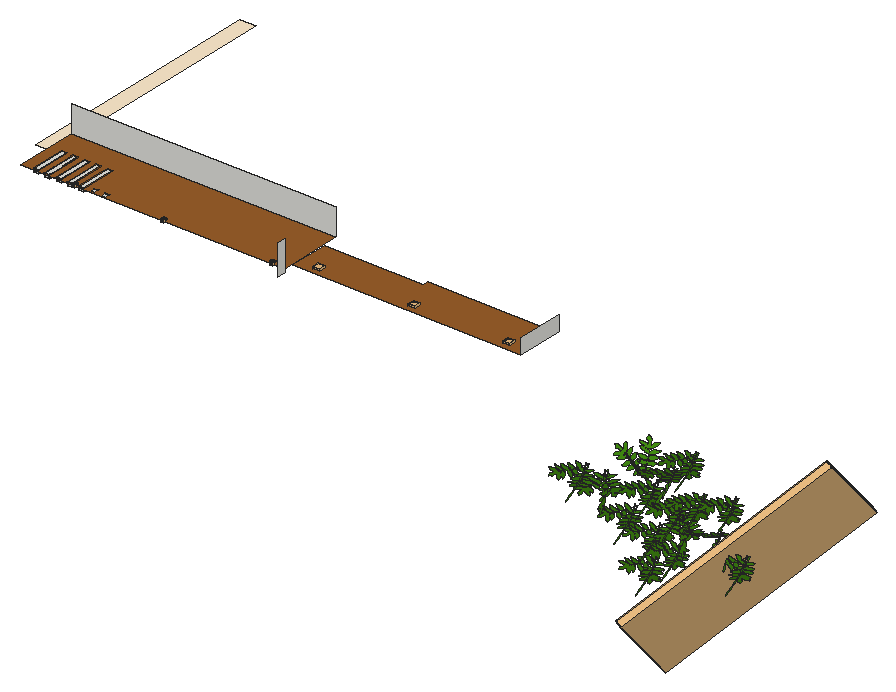
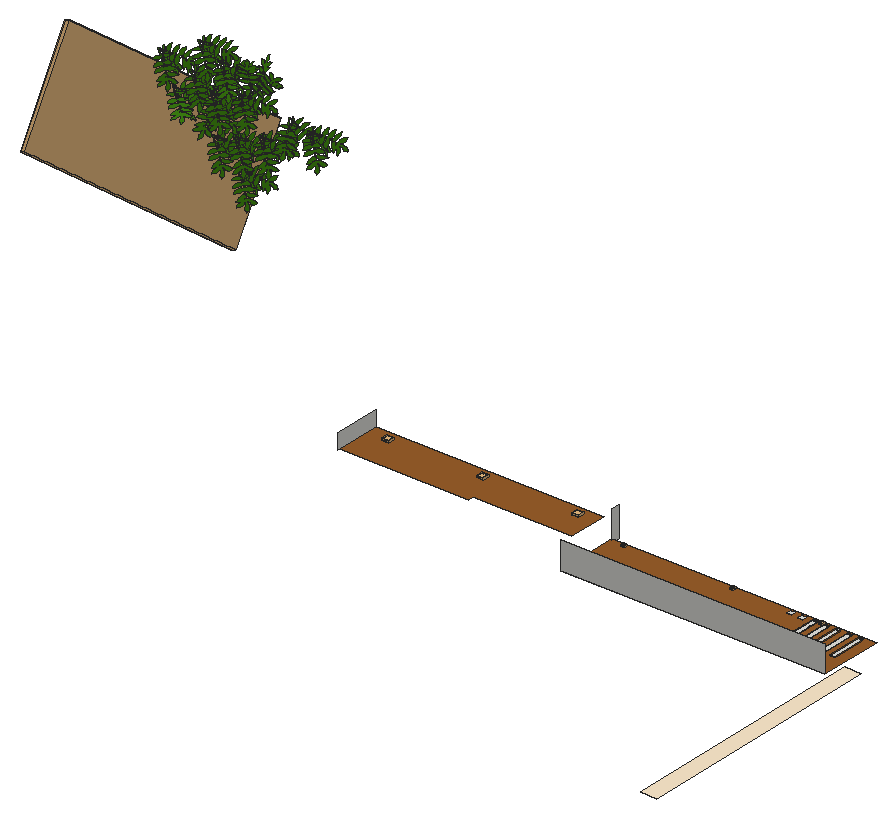
# SketchUp Ruby script. Lengths in inches.
U = 1.inch
M = Sketchup.active_model
def pt(a) = Geom::Point3d.new(a.map { |v| v * U })
def face(e, loops, mat)
  f = e.add_face(loops[0].map { |a| pt(a) })
  loops[1..].each { |l| e.add_face(l.map { |a| pt(a) }).erase! }
  f.material = f.back_material = mat if mat
  f
end
# faces: each face lists its corners as indices into pts; further lists are holes
def faces(e, pts, list, mat = nil) = list.each { |f| face(e, (f[0].is_a?(Array) ? f : [f]).map { |l| l.map { |i| pts[i] } }, mat) }
# xy, xz, yz: faces in a plane at the given z, y or x. An outline is a flat list of corners, or four numbers for a rectangle; further outlines are holes
def ring(l) = l.size == 4 ? [[l[0], l[1]], [l[2], l[1]], [l[2], l[3]], [l[0], l[3]]] : l.each_slice(2).to_a
def flat(e, list, mat, &to3) = list.each { |f| face(e, (f[0].is_a?(Array) ? f : [f]).map { |l| ring(l).map { |u, v| to3.(u, v) } }, mat) }
def xy(e, z, list, mat = nil) = flat(e, list, mat) { |x, y| [x, y, z] }
def xz(e, y, list, mat = nil) = flat(e, list, mat) { |x, z| [x, y, z] }
def yz(e, x, list, mat = nil) = flat(e, list, mat) { |y, z| [x, y, z] }
def lines(e, pts, list) = list.each { |a, b| e.add_line(pt(pts[a]), pt(pts[b])) }
# prism: a flat outline (further loops are holes) pulled along v
def prism(e, loops, v, mat = nil)
  f = face(e, loops, mat); d = Geom::Vector3d.new(v.map { |x| x * U })
  f.pushpull(f.normal.samedirection?(d) ? d.length : -d.length)
end
def box(e, o, s, mat = nil) = prism(e, [[o, [o[0] + s[0], o[1], o[2]], [o[0] + s[0], o[1] + s[1], o[2]], [o[0], o[1] + s[1], o[2]]]], [0, 0, s[2]], mat)
def at(x, y, z, deg = 0) = Geom::Transformation.translation(pt([x, y, z])) * Geom::Transformation.rotation(ORIGIN, Z_AXIS, deg.degrees)
def axes(o, x, y, z) = Geom::Transformation.new([*x, 0, *y, 0, *z, 0, *pt(o).to_a, 1])
def part(name) = M.definitions.add(name)
# library, detail: a bought-in or finely detailed component or shape, given as its bounding box
def library(name, o, s) = part(name).tap { |d| box(d.entities, o, s) }
def detail(e, o, s) = box(e.add_group.entities, o, s)
def put(e, d, t, mat = nil) = e.add_instance(d, t).tap { |i| i.material = mat if mat }
def group(e, t, mat = nil) = e.add_group.tap { |g| g.transformation = t; g.material = mat if mat }.entities
root = M.entities
M.materials.add("[0029_BlanchedAlmond]").color = [255, 235, 205]
M.materials.add("[Wood Floor Dark]").color = [153, 94, 42]
M.materials.add("hojas").color = [70, 150, 19]
c1 = library("Group\#88",[0,0,0],[77.52,5,145.33])
c2 = library("A$C06767DEF\#1",[-8.3,1.21,0],[7.09,7.09,5.51])
c3 = part("rama-acacia")
p = [[-13.53,0.69,-1.07],[-13.38,0.86,-0.98],[-13.61,0.85,-1.06],[-14.07,0.85,-1.21],[-15.17,0.86,-1.58],[-15.95,0.92,-1.83],
  [-16.01,1,-1.83],[-16.01,1.17,-1.78],[-16.07,1.93,-1.6],[-16.4,2.73,-1.5],[-16.65,3.06,-1.5],[-17.13,4.01,-1.41],
  [-17.78,4.7,-1.44],[-18.28,5.07,-1.51],[-18.57,5.18,-1.58],[-18.91,5.47,-1.62],[-19.07,5.48,-1.67],[-19.35,5.61,-1.73],
  [-19.51,5.64,-1.78],[-19.38,5.57,-1.75],[-19.33,5.5,-1.75],[-19.31,5.23,-1.82],[-19.38,5.08,-1.89],[-19.41,4.84,-1.96],
  [-19.36,4.59,-2.01],[-19.43,4.55,-2.04],[-19.36,4.15,-2.125],[-19.21,3.7,-2.19],[-18.875,3.1,-2.24],[-18.61,2.78,-2.24],
  [-17.83,2.19,-2.13],[-17.4375,1.85,-2.09],[-17.04,1.49,-2.05],[-16.61,1.24,-1.97],[-16.17,1.0625,-1.87],[-16.06,0.95,-1.86],
  [-16.06,0.91,-1.87],[-16.32,0.9,-1.96],[-16.7,0.88,-2.1],[-17.05,0.91,-2.21],[-17.61,1.15,-2.33],[-18.06,1.29,-2.45],
  [-18.88,1.53,-2.67],[-20.25,1.46,-3.15],[-20.59,1.49,-3.26],[-20.79,1.37,-3.36],[-21.08,1.2,-3.5],[-21.28,1.22,-3.5625],
  [-21.48,0.94,-3.71],[-21.79,0.5,-3.93],[-22.02,0.17,-4.1],[-22.11,0.05,-4.16],[-22.21,-0.02,-4.21],[-22.375,-0.05,-4.28],
  [-22.375,-0.07,-4.28],[-22.18,-0.09,-4.22],[-22.11,-0.07,-4.19],[-21.78,-0.1,-4.09],[-21.6,-0.18,-4.05],[-21.52,-0.27,-4.04],
  [-21.33,-0.33,-4],[-20.94,-0.54,-3.92],[-20.6875,-0.63,-3.86],[-20.54,-0.68,-3.82],[-20.42,-0.67,-3.78],[-20.09,-0.46,-3.61],
  [-19.8,-0.24,-3.45],[-19.21,-0.02,-3.19],[-18.48,0.08,-2.92],[-17.72,0.38,-2.58],[-17.4,0.5,-2.4375],[-16.93,0.75,-2.21],
  [-16.78,0.8,-2.15],[-16.1,0.83,-1.91],[-16.0625,0.81,-1.9],[-16.08,0.77,-1.91],[-16.27,0.72,-1.99],[-16.88,0.39,-2.29],
  [-17.1875,0.15,-2.46],[-17.27,0.02,-2.52],[-17.94,-0.52,-2.89],[-17.94,-0.59,-2.91],[-18.08,-0.68,-2.99],[-18.13,-0.86,-3.05],
  [-18.56,-1.55,-3.38],[-18.71,-2.11,-3.58],[-18.79,-2.61,-3.74],[-18.86,-2.84,-3.83],[-18.87,-3.07,-3.89],[-18.84,-3.22,-3.92],
  [-18.8,-3.26,-3.92],[-18.76,-3.47,-3.96],[-18.76,-3.6,-4],[-18.67,-3.8,-4.02],[-18.61,-3.92,-4.04],[-18.58,-4.11,-4.07],
  [-18.53,-4.18,-4.08],[-18.58,-4.35,-4.14],[-18.65,-4.43,-4.18],[-18.72,-4.51,-4.23],[-18.8125,-4.51,-4.26],[-18.8125,-4.53,-4.26],
  [-18.72,-4.54,-4.24],[-18.66,-4.49,-4.21],[-18.58,-4.43,-4.16],[-18.35,-4.23,-4.03],[-18.32,-4.17,-4],[-18.22,-4.125,-3.95],
  [-18.1,-4,-3.88],[-17.79,-3.72,-3.7],[-17.68,-3.51,-3.61],[-17.32,-3.13,-3.38],[-17.24,-2.94,-3.31],[-16.78,-2.12,-2.93],
  [-16.48,-1.78,-2.73],[-16.3,-1.28,-2.54],[-16.05,-0.75,-2.3125],[-15.89,-0.2,-2.11],[-15.89,0.39,-1.95],[-15.96,0.79,-1.87],
  [-15.91,0.82,-1.84],[-15.27,0.8,-1.63],[-14.18,0.76,-1.27],[-13.78,0.73,-1.15],[-13.78,0.67,-1.16],[-14.23,0.54,-1.35],
  [-14.65,0.33,-1.55],[-14.97,0.02,-1.74],[-15.25,-0.36,-1.9375],[-15.57,-0.72,-2.14],[-15.96,-1.64,-2.52],[-16.2,-2.51,-2.84],
  [-16.2,-3.12,-3],[-16.14,-3.41,-3.06],[-16.1,-3.75,-3.14],[-16.1,-4.09,-3.23],[-16.2,-4.25,-3.3],[-16.2,-4.28,-3.3125],
  [-16.08,-4.19,-3.24],[-15.98,-4.08,-3.18],[-15.96,-3.94,-3.14],[-15.96,-3.8125,-3.1],[-15.9,-3.72,-3.06],[-15.68,-3.55,-2.9375],
  [-15.51,-3.49,-2.86],[-15.3,-3.33,-2.75],[-15.23,-3.17,-2.68],[-15.01,-3.03,-2.57],[-14.875,-2.83,-2.47],[-14.6,-2.59,-2.3125],
  [-14.4,-2.27,-2.16],[-14.12,-1.6,-1.89],[-13.91,-1.1,-1.68],[-13.67,-0.83,-1.53],[-13.53,-0.45,-1.38],[-13.53,0.67,-1.08],
  [-12.41,6.01,0.65],[-12.44,6.14,0.68],[-12.41,6.29,0.73],[-12.43,6.29,0.73],[-12.44,6.26,0.72],[-12.47,6.15,0.68],
  [-12.49,6.07,0.66],[-12.57,5.75,0.55],[-12.67,5.36,0.43],[-12.79,4.875,0.28],[-12.83,4.52,0.18],[-12.83,3.99,0.04],
  [-12.73,3.11,-0.18],[-12.58,2.52,-0.3125],[-12.3,1.97,-0.41],[-11.88,1.51,-0.46],[-11.37,1.0625,-0.48],[-10.75,0.75,-0.45],
  [-10.75,0.68,-0.47],[-12.55,0.7,-0.79],[-13.21,0.79,-0.89],[-13.2,0.67,-0.92],[-12.56,0.62,-0.82],[-11.15,0.56,-0.58],
  [-10.79,0.54,-0.52],[-10.72,0.52,-0.51],[-10.72,0.5,-0.52],[-10.87,0.47,-0.55],[-11.14,0.41,-0.62],[-11.39,0.27,-0.7],
  [-11.625,-0.01,-0.82],[-11.8,-0.43,-0.96],[-11.83,-0.57,-1],[-12.02,-1.08,-1.17],[-12.1,-1.39,-1.27],[-12.17,-1.95,-1.4375],
  [-12.17,-2.77,-1.65],[-12.09,-3.59,-1.86],[-11.86,-4.26,-2],[-11.8125,-4.4,-2.03],[-11.84,-4.49,-2.05],[-11.91,-4.6,-2.1],
  [-11.97,-4.65,-2.12],[-11.98,-4.67,-2.13],[-11.92,-4.65,-2.11],[-11.84,-4.59,-2.08],[-11.77,-4.52,-2.05],[-11.74,-4.47,-2.03],
  [-11.37,-4.3125,-1.92],[-10.95,-4.0625,-1.78],[-10.82,-3.89,-1.71],[-10.64,-3.57,-1.59],[-10.41,-3.05,-1.41],[-10.27,-2.73,-1.3],
  [-10.07,-1.88,-1.03],[-10.15,-0.71,-0.73],[-10.31,-0.1,-0.6],[-10.5,0.4,-0.5],[-10.5,0.48,-0.48],[-10.44,0.53,-0.45],
  [-10.39,0.64,-0.42],[-10.52,0.73,-0.42],[-10.44,0.93,-0.35],[-10.44,1.2,-0.28],[-10.32,1.47,-0.18],[-10.48,2.6875,0.12],
  [-10.43,2.96,0.2],[-10.75,3.87,0.38],[-11.26,4.93,0.57],[-11.8,5.54,0.64],[-12.37,5.93,0.64],[-7.78,0.19,-0.06],
  [-7.78,0.25,-0.04],[-7.75,0.39,0],[-7.89,0.4,-0.02],[-7.96,0.46,-0.02],[-7.96,0.49,-0.01],[-7.76,0.62,0.06],
  [-7.53,0.99,0.2],[-7.31,1.78,0.45],[-7.31,2.74,0.71],[-7.63,3.6875,0.9],[-8.02,4.57,1.07],[-8.66,5.23,1.13],
  [-8.83,5.4,1.14],[-8.92,5.54,1.16],[-9.1,5.64,1.16],[-9.08,5.6,1.15],[-9.02,5.56,1.15],[-8.94,5.46,1.14],
  [-8.9,5.37,1.12],[-8.9375,5.25,1.08],[-9.14,4.92,0.96],[-9.31,4.5625,0.83],[-9.39,3.73,0.6],[-9.44,2.76,0.32],
  [-9.23,1.59,0.05],[-8.82,0.9,-0.06],[-8.36,0.59,-0.0625],[-8.14,0.51,-0.04],[-8.05,0.48,-0.03],[-8.05,0.46,-0.04],
  [-8.12,0.43,-0.06],[-10.1,0.49,-0.4],[-8.22,0.3125,-0.11],[-8.22,0.25,-0.125],[-8.53,0.13,-0.21],[-8.8,-0.16,-0.34],
  [-8.96,-0.61,-0.49],[-8.96,-0.87,-0.56],[-9.16,-1.42,-0.74],[-9.13,-1.77,-0.83],[-9.09,-1.83,-0.84],[-9.125,-1.92,-0.87],
  [-9.125,-2.13,-0.93],[-9.08,-2.23,-0.95],[-9.15,-2.39,-1],[-9.11,-2.67,-1.07],[-9.03,-2.86,-1.11],[-9.07,-3.03,-1.16],
  [-8.97,-3.23,-1.19],[-8.93,-3.44,-1.24],[-8.93,-3.71,-1.32],[-8.79,-4.05,-1.38],[-8.7,-4.25,-1.42],[-8.7,-4.39,-1.46],
  [-8.76,-4.53,-1.5],[-8.77,-4.65,-1.54],[-8.64,-4.55,-1.49],[-8.27,-4.22,-1.33],[-8.1875,-4.06,-1.27],[-8.07,-3.98,-1.23],
  [-7.98,-3.79,-1.17],[-7.79,-3.59,-1.08],[-7.64,-3.3,-0.97],[-7.64,-3.25,-0.96],[-7.59,-3.21,-0.9375],[-7.52,-2.93,-0.85],
  [-7.52,-2.85,-0.83],[-7.47,-2.81,-0.81],[-7.3,-2.09,-0.59],[-7.32,-2.01,-0.57],[-7.27,-1.95,-0.54],[-7.1875,-1.57,-0.42],
  [-7.17,-1.46,-0.39],[-7.17,-1.16,-0.3125],[-7.23,-0.61,-0.17],[-7.49,-0.15,-0.1],[-13.39,-0.07,-1.23],[-13.39,0.25,-1.14],
  [-13.49,0.5625,-1.09],[-13.8,1.01,-1.08],[-13.61,0.91,-1.04],[-13.38,0.92,-0.96],[-13.32,1.03,-0.91],[-13.32,1.35,-0.82],
  [-13.28,1.49,-0.77],[-13.28,1.99,-0.64],[-13.44,2.67,-0.51],[-13.72,3.31,-0.43],[-13.93,3.71,-0.4],[-14.1,4.39,-0.27],
  [-14.5625,5.06,-0.25],[-14.89,5.62,-0.21],[-15.33,6.1,-0.23],[-15.65,6.8,-0.15],[-15.79,6.89,-0.18],[-15.61,6.52,-0.22],
  [-15.51,6.32,-0.24],[-15.45,6.28,-0.23],[-15.52,6,-0.32],[-15.63,5.6875,-0.45],[-15.77,4.97,-0.68],[-15.7,4.25,-0.85],
  [-15.46,3,-1.11],[-15,2.03,-1.21],[-14.3,1.29,-1.17],[-4.5625,0.33,0.09],[-4.22,0.49,0.13],[-4,0.7,0.1875],
  [-3.86,0.99,0.26],[-3.77,1.41,0.38],[-3.7,1.73,0.46],[-3.77,1.99,0.53],[-3.85,2.17,0.58],[-3.88,2.57,0.6875],
  [-3.98,2.9,0.78],[-4.0625,2.97,0.8],[-4.1,3.14,0.84],[-4.1875,3.25,0.87],[-4.27,3.55,0.95],[-4.31,3.71,0.99],
  [-4.42,3.9,1.04],[-4.625,4.2,1.125],[-4.72,4.39,1.18],[-4.89,4.57,1.23],[-4.98,4.73,1.27],[-5,4.72,1.26],
  [-5.01,4.51,1.21],[-4.96,4.32,1.16],[-4.97,4.27,1.14],[-5.14,3.78,1.01],[-5.3,3.39,0.91],[-5.44,2.76,0.74],
  [-5.5,2.09,0.56],[-5.57,1.78,0.48],[-5.57,1.42,0.38],[-5.57,1.09,0.29],[-5.47,0.72,0.19],[-5.22,0.44,0.12],
  [-4.93,0.27,0.07],[-4.76,0.22,0.06],[-4.76,0.18,0.05],[-4.83,0.16,0.04],[-5.26,0,0],[-5.34,-0.04,-0.01],
  [-5.47,-0.22,-0.06],[-5.51,-0.6,-0.16],[-5.42,-1.09,-0.29],[-5.28,-1.49,-0.4],[-5.21,-1.87,-0.5],[-5.11,-2.15,-0.57],
  [-5.08,-2.34,-0.63],[-5.01,-2.47,-0.66],[-4.96,-2.69,-0.72],[-4.86,-2.9375,-0.79],[-4.84,-3.07,-0.82],[-4.77,-3.18,-0.85],
  [-4.74,-3.43,-0.92],[-4.7,-3.71,-0.99],[-4.62,-3.89,-1.04],[-4.58,-3.98,-1.07],[-4.58,-3.83,-1.03],[-4.51,-3.67,-0.98],
  [-4.3,-3.32,-0.89],[-4.16,-3.09,-0.83],[-4.16,-2.98,-0.8],[-4.11,-2.92,-0.78],[-4.02,-2.8,-0.75],[-3.95,-2.59,-0.69],
  [-3.95,-2.33,-0.625],[-3.86,-2.26,-0.6],[-3.86,-2.02,-0.54],[-3.86,-1.44,-0.39],[-3.94,-1.22,-0.33],[-3.94,-1.08,-0.29],
  [-4,-0.96,-0.26],[-4,-0.87,-0.23],[-4.0625,-0.8125,-0.22],[-4.16,-0.54,-0.14],[-4.39,-0.24,-0.06],[-4.61,-0.08,-0.02],
  [-4.77,-0.03,-0.01],[-4.77,-0.01,0],[-4.65,-0.01,0],[-4.61,0.19,0.05],[-4.66,0.23,0.0625],[-4.63,0.29,0.08],
  [-4.07,0.17,0.04],[0,-0.24,-0.06],[0,0,0],[-0.5,0.04,0.01],[-1.58,0.08,0.02],[-13.78,0.67,-1.08]]
faces(c3.entities,p,[[0,1,2,3,4,5,6,7,8,9,10,11,12,13,14,15,16,17,18,19,20,21,22,23,24,25,26,27,28,29,30,31,32,33,34,35,36,37,38,39,40,41,42,43,44,45,46,47,48,49,50,51,52,53,54,55,56,57,58,59,60,61,62,63,64,65,66,67,68,69,70,71,72,73,74,75,76,77,78,79,80,81,82,83,84,85,86,87,88,89,90,91,92,93,94,95,96,97,98,99,100,101,102,103,104,105,106,107,108,109,110,111,112,113,114,115,116,117,118,119,120,121,122,123,124,125,126,127,128,129,130,131,132,133,134,135,136,137,138,139,140,141,142,143,144,145,146,147,148,149,150,151,152,153,154,155],[156,157,158,159,160,161,162,163,164,165,166,167,168,169,170,171,172,173,174,175,176,177,178,179,180,181,182,183,184,185,186,187,188,189,190,191,192,193,194,195,196,197,198,199,200,201,202,203,204,205,206,207,208,209,210,211,212,213,214,215,216,217,218,219,220,221,222,223,224,225,226],[227,228,229,230,231,232,233,234,235,236,237,238,239,240,241,242,243,244,245,246,247,248,249,250,251,252,253,254,255,256,257,258,216,215,259,260,261,262,263,264,265,266,267,268,269,270,271,272,273,274,275,276,277,278,279,280,281,282,283,284,285,286,287,288,289,290,291,292,293,294,295,296,297,298,299,300,301,302,303],[154,304,305,306,155],[307,308,1,309,310,311,312,313,314,315,316,317,318,319,320,321,322,323,324,325,326,327,328,329,330,331,332],[333,334,335,336,337,338,339,340,341,342,343,344,345,346,347,348,349,350,351,352,353,354,355,356,357,358,359,360,361,362,363,364,365,366,367,368,369,370,371,372,373,374,375,376,377,378,379,380,381,382,383,384,385,386,387,388,389,390,391,392,393,394,395,396,397,398,399,400,401,402,403,404,405,406,407,408,409,410,411,412,413],[0,177,1],[308,2,1],
  [176,1,177],[414,411,410,415,416,417,418],[228,370,229],[369,229,370]],"hojas")
lines(c3.entities,p,[[155,419]])
c4 = part("Group\#83")
put(c4.entities,c3,axes([10.13,10.27,0],[0.45315,0.21131,0],[-0.21131,0.45315,0],[0,0,0.5]))
put(c4.entities,c3,axes([10.13,10.27,0],[0.11638,0.47539,0.10227],[-0.48087,0.12813,-0.0484],[-0.07223,-0.08709,0.48703]))
put(c4.entities,c3,axes([9.58,10.26,-0.7],[0.1449,0.38901,-0.2787],[-0.10883,0.31035,0.37662],[0.46601,-0.04848,0.17461]))
c5 = part("Group\#84")
put(c5.entities,c4,axes([24.99,4.24,9.59],[0.78856,0.61496,0],[0.01473,-0.01889,0.99971],[0.61478,-0.78833,-0.02396]))
put(c5.entities,c4,axes([39.5,6.625,12.55],[0.6544,0.49291,0.57341],[-0.44023,-0.3682,0.81892],[0.61478,-0.78833,-0.02396]))
put(c5.entities,c4,axes([32.34,3.7,6.88],[0.78856,0.61496,0],[0.01473,-0.01889,0.99971],[0.61478,-0.78833,-0.02396]))
put(c5.entities,c4,axes([43.14,6.65,17.54],[0.78856,0.61496,0],[0.35273,-0.4523,0.81915],[0.50374,-0.64595,-0.57358]))
put(c5.entities,c4,axes([12.2,6.2,16.68],[0.7209,0.54936,0.4225],[-0.31991,-0.27701,0.90605],[0.61478,-0.78833,-0.02396]))
put(c5.entities,c4,axes([49.9375,3.79,26.09],[0.78856,0.61496,0],[0.01473,-0.01889,0.99971],[0.61478,-0.78833,-0.02396]))
put(c5.entities,c4,axes([36.11,4.9375,33.94],[0.78856,0.61496,0],[0.01473,-0.01889,0.99971],[0.61478,-0.78833,-0.02396]))
put(c5.entities,c4,axes([39.61,3.79,23.47],[0.78856,0.61496,0],[0.01473,-0.01889,0.99971],[0.61478,-0.78833,-0.02396]))
put(c5.entities,c4,axes([25.59,6.5625,46.47],[-0.40704,-0.29112,-0.86578],[0.67555,0.54201,-0.49986],[0.61478,-0.78833,-0.02396]))
put(c5.entities,c4,axes([54.97,1.98,11.65],[0.78856,0.61496,0],[0.01473,-0.01889,0.99971],[0.61478,-0.78833,-0.02396]))
put(c5.entities,c4,axes([32.97,3.79,19.14],[0.78856,0.61496,0],[0.01473,-0.01889,0.99971],[0.61478,-0.78833,-0.02396]))
put(c5.entities,c4,axes([24.24,3.79,21.99],[0.78856,0.61496,0],[0.01473,-0.01889,0.99971],[0.61478,-0.78833,-0.02396]))
put(c5.entities,c4,axes([16.86,4.24,12.3],[0.78856,0.61496,0],[0.01473,-0.01889,0.99971],[0.61478,-0.78833,-0.02396]))
put(c5.entities,c4,axes([1.23,3.9375,19.07],[0.78856,0.61496,0],[0.01473,-0.01889,0.99971],[0.61478,-0.78833,-0.02396]))
put(c5.entities,c4,axes([29.05,5.25,29.11],[0.78856,0.61496,0],[0.21033,-0.2697,0.93969],[0.57787,-0.741,-0.34202]))
put(c5.entities,c4,axes([24.16,3.79,-0.1],[0.78856,0.61496,0],[0.01473,-0.01889,0.99971],[0.61478,-0.78833,-0.02396]))
xy(root,253.6875,[[101.6875,440.22,118.89,712.1]],"[0029_BlanchedAlmond]")
xy(root,254.91,[[203.55,404.92,208.86,405.01]])
xy(root,254.91,[[130.43,401.21,135.74,431.86],[142.61,401.21,147.93,431.86],[154.8,401.21,160.11,431.86],[166.99,401.21,172.3,431.86],[179.18,401.21,184.49,431.86],
  [130.43,431.86,135.74,438.86],[142.61,431.86,147.93,438.86],[154.8,431.86,160.11,438.86],[166.99,431.86,172.3,438.86],[179.18,431.86,184.49,438.86]],"[Wood Floor Dark]")
xy(root,258.66,[[130.43,399.67,135.74,401.21],[142.61,399.67,147.93,401.21],[154.8,399.67,157.63,399.67,160.11,401.21,154.8,401.21],[157.63,399.67,160.11,401.21,160.11,399.67],[166.99,399.67,172.3,401.21],
  [179.18,399.67,184.49,401.21],[191.36,399.67,196.68,405.64],[203.55,399.67,208.86,404.92],[130.43,401.21,135.74,438.86],[142.61,401.21,147.93,438.86],
  [154.8,401.21,160.11,438.86],[166.99,401.21,172.3,438.86],[179.18,401.21,184.49,438.86]])
xy(root,258.66,[[[118.89,397.92,400.76,466.49],[154.8,399.67,160.11,438.86],[166.99,399.67,172.3,438.86],[130.43,399.67,135.74,438.86],[142.61,399.67,147.93,438.86],[179.18,399.67,184.49,438.86],[191.36,399.67,196.68,405.64],[203.55,399.67,208.86,404.92],[269.98,398.5625,270.5,398.61,271,398.79,271.42,399.09,271.76,399.49,271.98,399.96,272.07,400.48,272.02,401,271.84,401.49,271.54,401.91,271.14,402.25,270.67,402.47,270.15,402.56,269.63,402.51,269.14,402.33,268.71,402.03,268.38,401.63,268.16,401.16,268.07,400.64,268.12,400.125,268.3,399.63,268.6,399.21,269,398.87,269.47,398.65],[386.05,398.5625,386.57,398.61,387.06,398.79,387.48,399.09,387.82,399.49,388.04,399.96,388.13,400.48,388.08,401,387.9,401.49,387.6,401.91,387.2,402.25,386.73,402.47,386.21,402.56,385.69,402.51,385.2,402.33,384.78,402.03,384.44,401.63,384.22,401.16,384.13,400.64,384.18,400.125,384.36,399.63,384.66,399.21,385.06,398.87,385.53,398.65],[174.67,398.5625,175.19,398.61,175.68,398.79,176.11,399.09,176.44,399.49,176.66,399.96,176.75,400.48,176.71,401,176.53,401.49,176.23,401.91,175.83,402.25,175.35,402.47,174.84,402.56,174.32,402.51,173.83,402.33,173.4,402.03,173.07,401.63,172.85,401.16,172.76,400.64,172.8,400.125,172.98,399.63,173.28,399.21,173.68,398.87,174.16,398.65]]],"[Wood Floor Dark]")
xy(root,259.66,[[174.67,398.5625,174.16,398.65,173.68,398.87,173.28,399.21,172.98,399.63,172.8,400.125,172.76,400.64,172.85,401.16,173.07,401.63,173.4,402.03,173.83,402.33,174.32,402.51,174.84,402.56,175.35,402.47,175.83,402.25,176.23,401.91,176.53,401.49,176.71,401,176.75,400.48,176.66,399.96,176.44,399.49,176.11,399.09,175.68,398.79,175.19,398.61],[269.98,398.5625,269.47,398.65,269,398.87,268.6,399.21,268.3,399.63,268.12,400.125,268.07,400.64,268.16,401.16,268.38,401.63,268.71,402.03,269.14,402.33,269.63,402.51,270.15,402.56,270.67,402.47,271.14,402.25,271.54,401.91,271.84,401.49,272.02,401,272.07,400.48,271.98,399.96,271.76,399.49,271.42,399.09,271,398.79,270.5,398.61],[386.05,398.5625,385.53,398.65,385.06,398.87,384.66,399.21,384.36,399.63,384.18,400.125,384.13,400.64,384.22,401.16,384.44,401.63,384.78,402.03,385.2,402.33,385.69,402.51,386.21,402.56,386.73,402.47,387.2,402.25,387.6,401.91,387.9,401.49,388.08,401,388.13,400.48,388.04,399.96,387.82,399.49,387.48,399.09,387.06,398.79,386.57,398.61]])
xy(root,271.24,[[436.55,397.34,435.75,397.45,435.02,397.75,434.38,398.24,433.89,398.875,433.59,399.61,433.48,400.4,433.59,401.2,433.89,401.9375,434.38,402.57,435.02,403.06,435.75,403.36,436.55,403.47,437.34,403.36,438.08,403.06,438.71,402.57,439.2,401.9375,439.5,401.2,439.61,400.4,439.5,399.61,439.2,398.875,438.71,398.24,438.08,397.75,437.34,397.45]])
xy(root,271.24,[[[416.52,389.67,416.52,431.86,522.24,431.86,522.24,437.41,660.05,437.41,660.05,389.67],[436.55,397.34,437.34,397.45,438.08,397.75,438.71,398.24,439.2,398.875,439.5,399.61,439.61,400.4,439.5,401.2,439.2,401.9375,438.71,402.57,438.08,403.06,437.34,403.36,436.55,403.47,435.75,403.36,435.02,403.06,434.38,402.57,433.89,401.9375,433.59,401.2,433.48,400.4,433.59,399.61,433.89,398.875,434.38,398.24,435.02,397.75,435.75,397.45],[537.75,397.34,538.54,397.45,539.28,397.75,539.92,398.24,540.4,398.875,540.71,399.61,540.8125,400.4,540.71,401.2,540.4,401.9375,539.92,402.57,539.28,403.06,538.54,403.36,537.75,403.47,536.96,403.36,536.22,403.06,535.59,402.57,535.1,401.9375,534.79,401.2,534.6875,400.4,534.79,399.61,535.1,398.875,535.59,398.24,536.22,397.75,536.96,397.45],[638.61,397.34,639.4,397.45,640.14,397.75,640.77,398.24,641.26,398.875,641.57,399.61,641.67,400.4,641.57,401.2,641.26,401.9375,640.77,402.57,640.14,403.06,639.4,403.36,638.61,403.47,637.82,403.36,637.08,403.06,636.44,402.57,635.96,401.9375,635.65,401.2,635.55,400.4,635.65,399.61,635.96,398.875,636.44,398.24,637.08,397.75,637.82,397.45]]],"[Wood Floor Dark]")
xz(root,401.21,[[130.43,254.91,135.74,258.66],[142.61,254.91,147.93,258.66],[154.8,254.91,160.11,258.66],[166.99,254.91,172.3,258.66],[179.18,254.91,184.49,258.66]])
xz(root,404.92,[[203.55,254.91,208.86,258.66]])
xz(root,405.64,[[191.36,254.91,196.68,258.66]])
xz(root,438.86,[[130.43,254.91,135.74,258.66],[142.61,254.91,147.93,258.66],[154.8,254.91,160.11,258.66]])
xz(root,438.86,[[166.99,254.91,172.3,258.66],[179.18,254.91,184.49,258.66]],"[Wood Floor Dark]")
xz(root,466.49,[[118.89,258.66,400.76,287.5625]])
yz(root,130.43,[[401.21,254.91,431.86,258.66],[431.86,254.91,438.86,258.66]],"[Wood Floor Dark]")
yz(root,135.74,[[401.21,254.91,431.86,258.66],[431.86,254.91,438.86,258.66]],"[Wood Floor Dark]")
yz(root,142.61,[[401.21,254.91,431.86,258.66],[431.86,254.91,438.86,258.66]],"[Wood Floor Dark]")
yz(root,147.93,[[401.21,254.91,431.86,258.66],[431.86,254.91,438.86,258.66]],"[Wood Floor Dark]")
yz(root,154.8,[[401.21,254.91,431.86,258.66],[431.86,254.91,438.86,258.66]],"[Wood Floor Dark]")
yz(root,160.11,[[401.21,254.91,431.86,258.66],[431.86,254.91,438.86,258.66]],"[Wood Floor Dark]")
yz(root,166.99,[[401.21,254.91,431.86,258.66],[431.86,254.91,438.86,258.66]],"[Wood Floor Dark]")
yz(root,172.3,[[401.21,254.91,431.86,258.66],[431.86,254.91,438.86,258.66]],"[Wood Floor Dark]")
yz(root,179.18,[[401.21,254.91,431.86,258.66],[431.86,254.91,438.86,258.66]],"[Wood Floor Dark]")
yz(root,184.49,[[401.21,254.91,431.86,258.66],[431.86,254.91,438.86,258.66]],"[Wood Floor Dark]")
yz(root,400.76,[[389.67,254.91,397.92,287.5625]])
yz(root,660.05,[[389.67,271.24,440.22,287.5625]])
p = [[174.67,398.5625,258.66],[174.16,398.65,258.66],[174.16,398.65,259.66],[174.67,398.5625,259.66],[175.19,398.61,258.66],[175.19,398.61,259.66],
  [175.68,398.79,258.66],[175.68,398.79,259.66],[269.98,398.5625,258.66],[269.47,398.65,258.66],[269.47,398.65,259.66],[269.98,398.5625,259.66],
  [270.5,398.61,258.66],[270.5,398.61,259.66],[271,398.79,258.66],[271,398.79,259.66],[386.05,398.5625,258.66],[385.53,398.65,258.66],
  [385.53,398.65,259.66],[386.05,398.5625,259.66],[386.57,398.61,258.66],[386.57,398.61,259.66],[387.06,398.79,258.66],[387.06,398.79,259.66],
  [173.68,398.87,258.66],[173.68,398.87,259.66],[269,398.87,258.66],[269,398.87,259.66],[385.06,398.87,258.66],[385.06,398.87,259.66],
  [176.11,399.09,258.66],[176.11,399.09,259.66],[271.42,399.09,258.66],[271.42,399.09,259.66],[387.48,399.09,258.66],[387.48,399.09,259.66],
  [173.28,399.21,258.66],[173.28,399.21,259.66],[268.6,399.21,258.66],[268.6,399.21,259.66],[384.66,399.21,258.66],[384.66,399.21,259.66],
  [176.44,399.49,258.66],[176.44,399.49,259.66],[271.76,399.49,258.66],[271.76,399.49,259.66],[387.82,399.49,258.66],[387.82,399.49,259.66],
  [172.98,399.63,258.66],[172.98,399.63,259.66],[268.3,399.63,258.66],[268.3,399.63,259.66],[384.36,399.63,258.66],[384.36,399.63,259.66],
  [176.66,399.96,258.66],[176.66,399.96,259.66],[271.98,399.96,258.66],[271.98,399.96,259.66],[388.04,399.96,258.66],[388.04,399.96,259.66],
  [172.8,400.125,258.66],[172.8,400.125,259.66],[268.12,400.125,258.66],[268.12,400.125,259.66],[384.18,400.125,258.66],[384.18,400.125,259.66],
  [176.75,400.48,258.66],[176.75,400.48,259.66],[272.07,400.48,258.66],[272.07,400.48,259.66],[388.13,400.48,258.66],[388.13,400.48,259.66],
  [172.76,400.64,258.66],[172.76,400.64,259.66],[268.07,400.64,258.66],[268.07,400.64,259.66],[384.13,400.64,258.66],[384.13,400.64,259.66],
  [176.71,401,258.66],[176.71,401,259.66],[272.02,401,258.66],[272.02,401,259.66],[388.08,401,258.66],[388.08,401,259.66],
  [172.85,401.16,258.66],[172.85,401.16,259.66],[268.16,401.16,258.66],[268.16,401.16,259.66],[384.22,401.16,258.66],[384.22,401.16,259.66],
  [176.53,401.49,258.66],[176.53,401.49,259.66],[271.84,401.49,258.66],[271.84,401.49,259.66],[387.9,401.49,258.66],[387.9,401.49,259.66],
  [173.07,401.63,258.66],[173.07,401.63,259.66],[268.38,401.63,258.66],[268.38,401.63,259.66],[384.44,401.63,258.66],[384.44,401.63,259.66],
  [176.23,401.91,258.66],[176.23,401.91,259.66],[271.54,401.91,258.66],[271.54,401.91,259.66],[387.6,401.91,258.66],[387.6,401.91,259.66],
  [173.4,402.03,258.66],[173.4,402.03,259.66],[268.71,402.03,258.66],[268.71,402.03,259.66],[384.78,402.03,258.66],[384.78,402.03,259.66],
  [175.83,402.25,258.66],[175.83,402.25,259.66],[271.14,402.25,258.66],[271.14,402.25,259.66],[387.2,402.25,258.66],[387.2,402.25,259.66],
  [173.83,402.33,258.66],[173.83,402.33,259.66],[269.14,402.33,258.66],[269.14,402.33,259.66],[385.2,402.33,258.66],[385.2,402.33,259.66],
  [175.35,402.47,258.66],[175.35,402.47,259.66],[270.67,402.47,258.66],[270.67,402.47,259.66],[386.73,402.47,258.66],[386.73,402.47,259.66],
  [174.32,402.51,258.66],[174.32,402.51,259.66],[269.63,402.51,258.66],[269.63,402.51,259.66],[385.69,402.51,258.66],[385.69,402.51,259.66],
  [174.84,402.56,258.66],[174.84,402.56,259.66],[270.15,402.56,258.66],[270.15,402.56,259.66],[386.21,402.56,258.66],[386.21,402.56,259.66],
  [537.75,397.34,271.24],[536.96,397.45,271.24],[536.96,397.45,272.11],[537.75,397.34,272.11],[538.54,397.45,271.24],[538.54,397.45,272.11],
  [638.61,397.34,271.24],[637.82,397.45,271.24],[637.82,397.45,272.11],[638.61,397.34,272.11],[639.4,397.45,271.24],[639.4,397.45,272.11],
  [536.22,397.75,271.24],[536.22,397.75,272.11],[539.28,397.75,271.24],[539.28,397.75,272.11],[637.08,397.75,271.24],[637.08,397.75,272.11],
  [640.14,397.75,271.24],[640.14,397.75,272.11],[535.59,398.24,271.24],[535.59,398.24,272.11],[539.92,398.24,271.24],[539.92,398.24,272.11],
  [636.44,398.24,271.24],[636.44,398.24,272.11],[640.77,398.24,271.24],[640.77,398.24,272.11],[535.1,398.875,271.24],[535.1,398.875,272.11],
  [540.4,398.875,271.24],[540.4,398.875,272.11],[635.96,398.875,271.24],[635.96,398.875,272.11],[641.26,398.875,271.24],[641.26,398.875,272.11],
  [534.79,399.61,271.24],[534.79,399.61,272.11],[540.71,399.61,271.24],[540.71,399.61,272.11],[635.65,399.61,271.24],[635.65,399.61,272.11],
  [641.57,399.61,271.24],[641.57,399.61,272.11],[534.6875,400.4,271.24],[534.6875,400.4,272.11],[540.8125,400.4,271.24],[540.8125,400.4,272.11],
  [635.55,400.4,271.24],[635.55,400.4,272.11],[641.67,400.4,271.24],[641.67,400.4,272.11],[534.79,401.2,271.24],[534.79,401.2,272.11],
  [540.71,401.2,271.24],[540.71,401.2,272.11],[635.65,401.2,271.24],[635.65,401.2,272.11],[641.57,401.2,271.24],[641.57,401.2,272.11],
  [535.1,401.9375,271.24],[535.1,401.9375,272.11],[540.4,401.9375,271.24],[540.4,401.9375,272.11],[635.96,401.9375,271.24],[635.96,401.9375,272.11],
  [641.26,401.9375,271.24],[641.26,401.9375,272.11],[535.59,402.57,271.24],[535.59,402.57,272.11],[539.92,402.57,271.24],[539.92,402.57,272.11],
  [636.44,402.57,271.24],[636.44,402.57,272.11],[640.77,402.57,271.24],[640.77,402.57,272.11],[536.22,403.06,271.24],[536.22,403.06,272.11],
  [539.28,403.06,271.24],[539.28,403.06,272.11],[637.08,403.06,271.24],[637.08,403.06,272.11],[640.14,403.06,271.24],[640.14,403.06,272.11],
  [536.96,403.36,271.24],[536.96,403.36,272.11],[538.54,403.36,271.24],[538.54,403.36,272.11],[637.82,403.36,271.24],[637.82,403.36,272.11],
  [639.4,403.36,271.24],[639.4,403.36,272.11],[537.75,403.47,271.24],[537.75,403.47,272.11],[638.61,403.47,271.24],[638.61,403.47,272.11]]
faces(root,p,[[0,1,2,3],[4,0,3,5],[6,4,5,7],[8,9,10,11],[12,8,11,13],[14,12,13,15],[16,17,18,19],[20,16,19,21],
  [22,20,21,23],[1,24,25,2],[9,26,27,10],[17,28,29,18],[30,6,7,31],[32,14,15,33],[34,22,23,35],[24,36,37,25],
  [26,38,39,27],[28,40,41,29],[42,30,31,43],[44,32,33,45],[46,34,35,47],[36,48,49,37],[38,50,51,39],[40,52,53,41],
  [54,42,43,55],[56,44,45,57],[58,46,47,59],[48,60,61,49],[50,62,63,51],[52,64,65,53],[66,54,55,67],[68,56,57,69],
  [70,58,59,71],[60,72,73,61],[62,74,75,63],[64,76,77,65],[78,66,67,79],[80,68,69,81],[82,70,71,83],[72,84,85,73],
  [74,86,87,75],[76,88,89,77],[90,78,79,91],[92,80,81,93],[94,82,83,95],[84,96,97,85],[86,98,99,87],[88,100,101,89],
  [102,90,91,103],[104,92,93,105],[106,94,95,107],[96,108,109,97],[98,110,111,99],[100,112,113,101],[114,102,103,115],[116,104,105,117],
  [118,106,107,119],[108,120,121,109],[110,122,123,111],[112,124,125,113],[126,114,115,127],[128,116,117,129],[130,118,119,131],[120,132,133,121],
  [122,134,135,123],[124,136,137,125],[132,138,139,133],[138,126,127,139],[134,140,141,135],[140,128,129,141],[136,142,143,137],[142,130,131,143],
  [144,145,146,147],[148,144,147,149],[150,151,152,153],[154,150,153,155],[145,156,157,146],[158,148,149,159],[151,160,161,152],[162,154,155,163],
  [156,164,165,157],[166,158,159,167],[160,168,169,161],[170,162,163,171],[164,172,173,165],[174,166,167,175],[168,176,177,169],[178,170,171,179],
  [172,180,181,173],[182,174,175,183],[176,184,185,177],[186,178,179,187],[180,188,189,181],[190,182,183,191],[184,192,193,185],[194,186,187,195],
  [188,196,197,189],[198,190,191,199],[192,200,201,193],[202,194,195,203],[196,204,205,197],[206,198,199,207],[200,208,209,201],[210,202,203,211],
  [204,212,213,205],[214,206,207,215],[208,216,217,209],[218,210,211,219],[212,220,221,213],[222,214,215,223],[216,224,225,217],[226,218,219,227],
  [220,228,229,221],[230,222,223,231],[224,232,233,225],[234,226,227,235],[228,236,237,229],[236,230,231,237],[232,238,239,233],[238,234,235,239]])
put(root,c1,axes([1010.75,137.9,207.16],[0.21554,-1.03818,1.08909],[1.32291,-0.3934,-0.63682],[0.71684,1.03818,0.84778]))
put(root,c2,axes([272.48,397.93,256.69],[0.525,0,0],[0,0.525,0],[0,0,0.525]))
put(root,c2,axes([388.54,397.93,256.69],[0.525,0,0],[0,0.525,0],[0,0,0.525]))
put(root,c2,axes([177.14,398.33,256.77],[0.525,0,0],[0,0.525,0],[0,0,0.525]))
put(root,c5,axes([888.3,123,264.24],[3.2832,0,0],[0,3.2832,0],[0,0,3.2832]))
put(root,c2,at(440.74,395.32,267.23))
put(root,c2,at(542.24,395.32,267.23))
put(root,c2,at(643.37,395.32,267.23))
